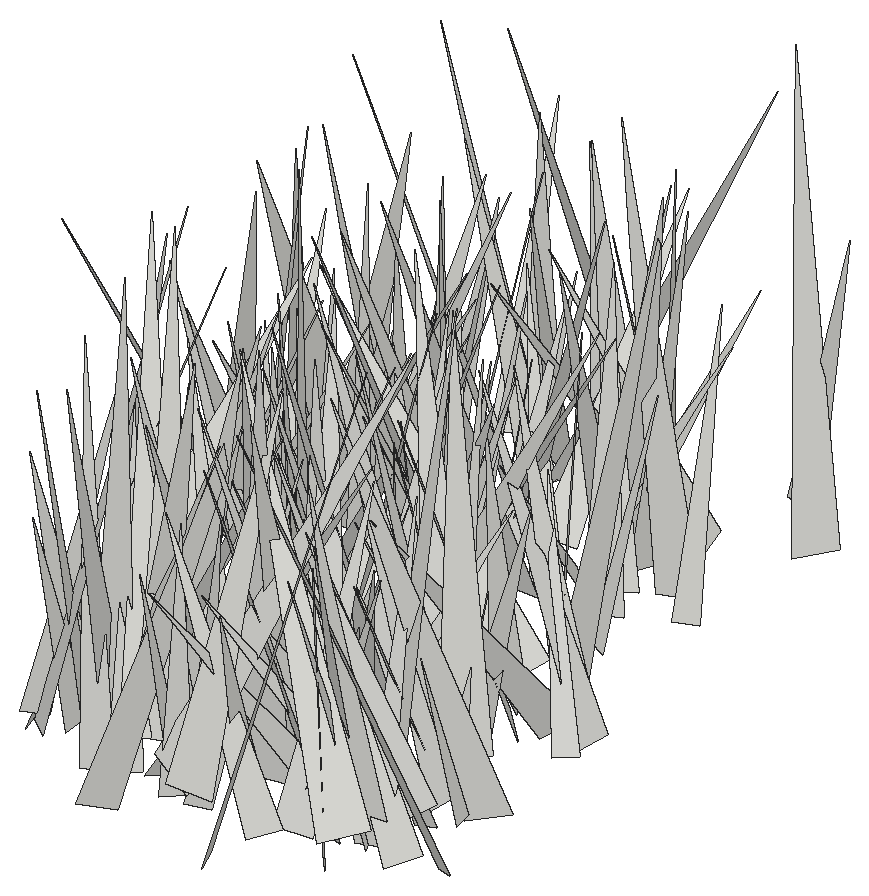
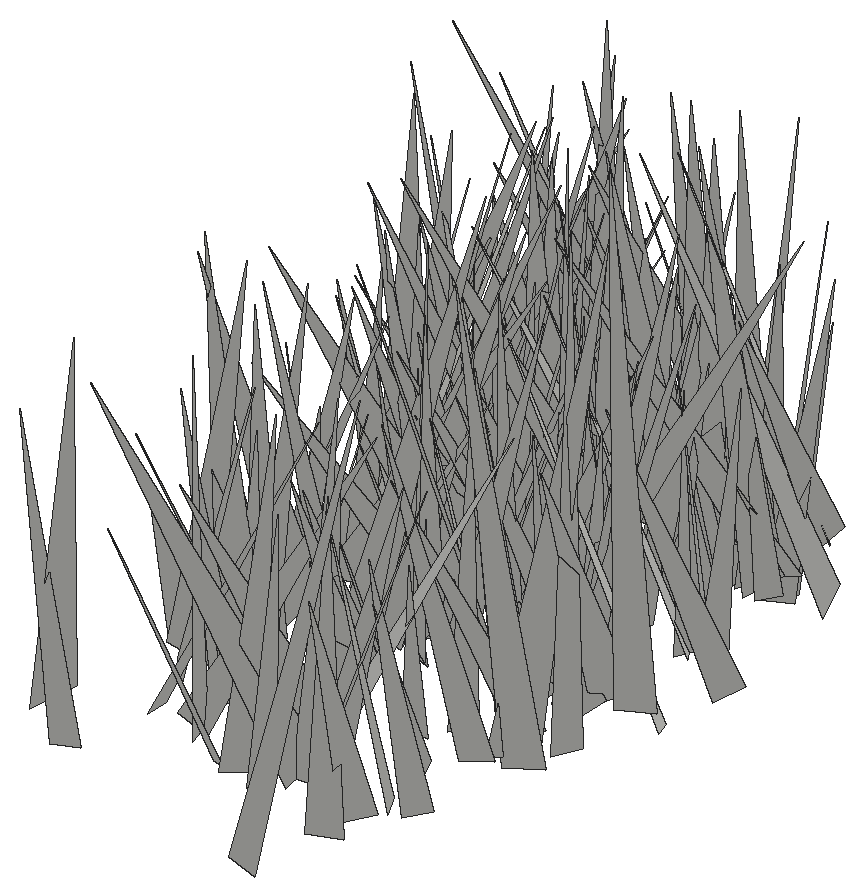
# SketchUp Ruby script. Lengths in inches.
U = 1.inch
M = Sketchup.active_model
def pt(a) = Geom::Point3d.new(a.map { |v| v * U })
def face(e, loops, mat)
  f = e.add_face(loops[0].map { |a| pt(a) })
  loops[1..].each { |l| e.add_face(l.map { |a| pt(a) }).erase! }
  f.material = f.back_material = mat if mat
  f
end
# faces: each face lists its corners as indices into pts; further lists are holes
def faces(e, pts, list, mat = nil) = list.each { |f| face(e, (f[0].is_a?(Array) ? f : [f]).map { |l| l.map { |i| pts[i] } }, mat) }
# xy, xz, yz: faces in a plane at the given z, y or x. An outline is a flat list of corners, or four numbers for a rectangle; further outlines are holes
def ring(l) = l.size == 4 ? [[l[0], l[1]], [l[2], l[1]], [l[2], l[3]], [l[0], l[3]]] : l.each_slice(2).to_a
def flat(e, list, mat, &to3) = list.each { |f| face(e, (f[0].is_a?(Array) ? f : [f]).map { |l| ring(l).map { |u, v| to3.(u, v) } }, mat) }
def xy(e, z, list, mat = nil) = flat(e, list, mat) { |x, y| [x, y, z] }
def xz(e, y, list, mat = nil) = flat(e, list, mat) { |x, z| [x, y, z] }
def yz(e, x, list, mat = nil) = flat(e, list, mat) { |y, z| [x, y, z] }
def lines(e, pts, list) = list.each { |a, b| e.add_line(pt(pts[a]), pt(pts[b])) }
# prism: a flat outline (further loops are holes) pulled along v
def prism(e, loops, v, mat = nil)
  f = face(e, loops, mat); d = Geom::Vector3d.new(v.map { |x| x * U })
  f.pushpull(f.normal.samedirection?(d) ? d.length : -d.length)
end
def box(e, o, s, mat = nil) = prism(e, [[o, [o[0] + s[0], o[1], o[2]], [o[0] + s[0], o[1] + s[1], o[2]], [o[0], o[1] + s[1], o[2]]]], [0, 0, s[2]], mat)
def at(x, y, z, deg = 0) = Geom::Transformation.translation(pt([x, y, z])) * Geom::Transformation.rotation(ORIGIN, Z_AXIS, deg.degrees)
def axes(o, x, y, z) = Geom::Transformation.new([*x, 0, *y, 0, *z, 0, *pt(o).to_a, 1])
def part(name) = M.definitions.add(name)
# library, detail: a bought-in or finely detailed component or shape, given as its bounding box
def library(name, o, s) = part(name).tap { |d| box(d.entities, o, s) }
def detail(e, o, s) = box(e.add_group.entities, o, s)
def put(e, d, t, mat = nil) = e.add_instance(d, t).tap { |i| i.material = mat if mat }
def group(e, t, mat = nil) = e.add_group.tap { |g| g.transformation = t; g.material = mat if mat }.entities
root = M.entities
c1 = part("fur_instance\#9")
p = [[0.8125,0,1.79],[0.67,-0.02,1.48],[0,-0.11,0],[0,0.11,0]]
faces(c1.entities,p,[[0,1,2,3]])
put(root,c1,axes([77.15,203.18,-28.22],[-4.827,3.94667,0.05385],[3.76525,4.62978,-1.80751],[1.18405,1.36675,5.96733]))
put(root,c1,axes([74.625,200.86,-28.22],[4.25693,-2.37845,0.80532],[-2.50825,-3.95225,1.586],[0.11926,1.77474,4.61119]))
put(root,c1,axes([74.94,208.11,-27.1],[7.73874,0.04549,1.82687],[0.5794,-7.60007,-2.26513],[-1.73315,-2.33761,7.39995]))
put(root,c1,axes([75.98,209.39,-27.1],[6.63906,-4.24471,1.17982],[-3.75911,-6.57064,-2.48644],[-2.29753,-1.51516,7.47745]))
put(root,c1,axes([76.89,193.25,-27.1],[-5.00496,1.9066,1.35129],[1.19771,4.83542,-2.3864],[2.00664,1.8693,4.79477]))
put(root,c1,axes([76.36,199.49,-28.22],[2.8154,-3.04723,0.70248],[-2.99803,-2.89898,-0.55973],[-0.88933,0.126,4.11081]))
put(root,c1,axes([77.24,215.06,-27.1],[-3.56448,3.67904,0.44666],[3.56023,3.5714,-1.00507],[1.02934,0.38746,5.02301]))
put(root,c1,axes([75.96,201.34,-27.1],[3.91592,-0.46866,0.80636],[-0.26131,-3.89224,-0.99321],[-0.89531,-0.91384,3.81675]))
put(root,c1,axes([76.02,199.99,-28.22],[3.95435,2.54343,1.52337],[2.80761,-4.0284,-0.56212],[-0.95239,-1.31514,4.66797]))
put(root,c1,axes([76.04,213.79,-27.1],[2.99214,-2.75371,1.44433],[-3.06357,-2.95389,0.71483],[-0.53251,1.52102,4.0031]))
put(root,c1,axes([77.03,195.6,-28.22],[3.57581,-3.48366,1.446],[-3.33217,-3.85124,-1.03819],[-1.76733,0.21279,4.88308]))
put(root,c1,axes([76.11,197.11,-27.1],[3.13443,-2.25979,0.73802],[-2.32723,-3.16608,0.18952],[-0.4851,0.5876,3.85946]))
put(root,c1,axes([80.1,201.87,-27.1],[-3.80092,-6.72254,0.0507],[-6.48684,3.65215,-2.05545],[-1.76524,1.05421,7.4441]))
put(root,c1,axes([74.91,204.93,-27.1],[-0.13317,-8.12567,1.45261],[-7.87911,0.55826,2.40046],[2.46092,1.34765,7.76415]))
put(root,c1,axes([80.11,213.3,-27.1],[-6.83624,-2.0461,0.45627],[-2.08301,6.45462,-2.26447],[-0.23611,2.29788,6.76704]))
put(root,c1,axes([77.03,195.1,-28.22],[3.88583,-1.17381,1.38743],[-0.79486,-4.04284,-1.19419],[-1.63432,-0.82466,3.87962]))
put(root,c1,axes([77.62,194.7,-27.1],[-4.6895,-2.45579,1.69505],[-2.43913,4.97359,0.45768],[1.71894,0.35769,5.27378]))
put(root,c1,axes([77.49,211.6,-27.1],[3.33394,1.47543,1.26624],[0.9738,-3.44268,1.44745],[-1.68284,0.93087,3.34618]))
put(root,c1,axes([75.34,209.65,-27.1],[0.9927,-7.18833,2.00129],[-7.23058,-0.4281,2.04891],[1.84279,2.19257,6.96128]))
put(root,c1,axes([81.21,210.83,-27.1],[-6.43148,-3.95381,0.27263],[-3.76371,5.93049,-2.78112],[-1.24153,2.50351,7.01869]))
put(root,c1,axes([76.65,196.6875,-27.1],[7.07212,-1.1156,2.41076],[-1.38462,-7.39913,0.63784],[-2.26697,1.03896,7.1311]))
put(root,c1,axes([79.22,193.26,-28.22],[0.02975,6.47261,1.15989],[6.34372,-0.33363,1.69906],[-1.73125,-1.11127,6.2457]))
put(root,c1,axes([77.39,216.53,-27.1],[1.77747,-4.94769,1.74658],[-5.22789,-1.82695,0.145],[-0.44649,1.69476,5.25529]))
put(root,c1,axes([78.15,205.01,-27.1],[0.81104,4.54834,1.26147],[4.65262,-0.98593,0.56355],[-0.7949,-1.13006,4.58559]))
put(root,c1,axes([79.71,201.18,-28.22],[-6.68615,-0.01766,0.93467],[0.01232,6.74773,0.2156],[0.93476,-0.21523,6.6827]))
put(root,c1,axes([78.14,219.46,-27.1],[-2.86218,-6.85746,0.77217],[-6.83354,2.93291,0.71683],[0.96112,0.43167,7.39614]))
put(root,c1,axes([78.36,203.05,-27.1],[-4.55771,-1.35516,1.4154],[-1.26006,4.77117,0.51063],[1.50069,-0.10962,4.72742]))
put(root,c1,axes([77.54,192.62,-27.1],[5.51307,6.12337,0.96272],[5.81555,-5.55551,2.03274],[-2.14519,0.67601,7.98483]))
put(root,c1,axes([76.74,208.48,-27.1],[1.64053,-3.56149,0.70323],[-3.59089,-1.47867,0.88831],[0.53314,0.99969,3.81922]))
put(root,c1,axes([76.97,213.89,-27.1],[4.26525,2.34746,1.0733],[2.44325,-4.34035,-0.2164],[-0.83252,-0.71113,4.86375]))
put(root,c1,axes([75.79,194.58,-28.22],[7.5502,3.19495,0.69372],[3.12341,-7.56468,0.84526],[-0.96605,0.51231,8.15468]))
put(root,c1,axes([76.69,210.18,-27.1],[-0.20342,5.45726,1.92359],[5.57072,0.70526,-1.41173],[1.56492,-1.80117,5.27542]))
put(root,c1,axes([79.24,201.59,-27.1],[-4.35702,1.54483,0.37411],[1.45493,4.3157,-0.87633],[0.64002,0.7059,4.53896]))
put(root,c1,axes([75.96,201.09,-27.1],[4.98455,3.49636,0.32674],[3.50629,-4.92427,-0.79656],[0.19289,-0.83908,6.03621]))
put(root,c1,axes([78.7,203.74,-28.22],[-4.7956,1.01448,1.55419],[0.95492,5.04106,-0.34401],[1.59148,0.0322,4.88965]))
put(root,c1,axes([78.79,198.26,-27.1],[-3.8802,0.07929,1.10053],[0.11582,4.03064,0.11798],[1.09728,-0.14508,3.87922]))
put(root,c1,axes([77.84,204.24,-28.22],[6.61822,-2.56323,1.80089],[-1.74555,-6.51281,-2.85492],[-2.60123,-2.15113,6.49773]))
put(root,c1,axes([74.86,203.72,-28.22],[5.8637,3.4963,0.04079],[3.31459,-5.53283,-2.23832],[1.11324,-1.94227,6.44958]))
put(root,c1,axes([76.23,208.14,-27.1],[4.34648,-1.55951,0.20323],[-1.53377,-4.07129,1.56122],[0.34774,1.53551,4.34586]))
put(root,c1,axes([79.76,213.33,-27.1],[0.51311,-4.91857,2.52241],[-5.22585,-1.25725,-1.38854],[-1.80151,2.24614,4.74633]))
put(root,c1,axes([79.17,210.01,-27.1],[-0.87591,3.86506,0.33078],[3.84564,0.82067,0.59405],[-0.50909,-0.4507,3.91829]))
put(root,c1,axes([76.67,195.89,-27.1],[-0.73588,7.38124,0.25307],[6.98236,0.77818,-2.39362],[2.40696,-0.00075,7.02103]))
put(root,c1,axes([78.65,201.09,-27.1],[5.2038,5.70361,2.35891],[5.67233,-5.63566,1.11317],[-2.43315,-0.93989,7.64013]))
put(root,c1,axes([78.25,208.86,-27.1],[4.81176,-1.3762,1.70282],[-1.26945,-5.10354,-0.53746],[-1.78382,-0.0803,4.97575]))
put(root,c1,axes([80.67,206.27,-27.1],[-3.32037,-5.8988,2.51801],[-6.36421,2.67847,-2.11746],[-0.7956,3.19234,6.42939]))
put(root,c1,axes([77.15,207.62,-27.1],[2.1882,-4.93746,0.79161],[-4.93819,-1.99768,1.19031],[0.78701,1.19336,5.26781]))
put(root,c1,axes([79.8125,204.48,-27.1],[1.26749,-5.25605,0.55346],[-5.00773,-1.37633,-1.60227],[-1.68968,0.13629,5.16385]))
put(root,c1,axes([78.76,194.54,-27.1],[-0.16128,6.84934,2.86842],[7.42417,0.20732,-0.07764],[0.15166,-2.86546,6.8508]))
put(root,c1,axes([78.35,195.32,-28.22],[6.75782,0.35235,2.65885],[1.16075,-6.88187,-2.03823],[-2.41791,-2.31896,6.45275]))
put(root,c1,axes([78.65,202.73,-28.22],[0.54293,-5.17192,1.62827],[-5.42158,-0.49338,0.24063],[0.08095,1.64396,5.19477]))
put(root,c1,axes([79.98,193.61,-28.22],[-5.05186,2.37101,0.85511],[2.22237,5.09377,-0.9944],[1.18912,0.55319,5.49128]))
put(root,c1,axes([80.45,194.16,-27.1],[-5.1988,6.07272,1.14347],[6.1224,5.26442,-0.12263],[0.83765,-0.78798,7.99315]))
put(root,c1,axes([79.75,199.91,-27.1],[-0.43977,4.5707,0.64422],[4.59918,0.3789,0.45132],[-0.39225,-0.6818,4.56957]))
put(root,c1,axes([77.23,204.14,-28.22],[5.25696,-1.00652,0.21452],[-1.02902,-5.15697,1.02054],[-0.01477,1.04274,5.25426]))
put(root,c1,axes([79.34,203.57,-28.22],[-4.01189,-2.17426,1.82805],[-1.57492,4.33524,1.69992],[2.36407,-0.80168,4.23473]))
put(root,c1,axes([80.69,197.24,-28.22],[-6.42976,0.15301,2.02637],[0.5172,6.6259,1.14077],[1.96522,-1.24316,6.3296]))
put(root,c1,axes([79.31,199.2,-28.22],[6.21031,-0.46369,2.15458],[0.49806,-5.98034,-2.72263],[-2.14689,-2.7287,5.60092]))
put(root,c1,axes([77.81,198.61,-27.1],[4.01839,-5.64573,1.18023],[-5.73753,-3.76564,1.52164],[0.58986,1.83314,6.76065]))
put(root,c1,axes([80.7,203.59,-27.1],[1.55743,6.34801,1.89562],[6.44853,-1.89902,1.06134],[-1.51893,-1.55328,6.44953]))
put(root,c1,axes([80.83,194.28,-27.1],[-1.87564,7.62096,1.95831],[7.8685,1.80971,0.49369],[-0.027,-2.0194,7.83284]))
put(root,c1,axes([80.94,215.03,-27.1],[-4.87312,1.26006,1.29377],[1.19613,5.04128,-0.40455],[1.35309,0.08157,5.01711]))
put(root,c1,axes([80.02,205.14,-28.22],[3.87453,3.49507,1.24049],[3.40824,-4.0629,0.80191],[-1.46226,-0.20898,5.15601]))
put(root,c1,axes([77.35,207.51,-27.1],[5.13352,5.29295,1.04527],[5.31008,-4.70157,-2.27141],[0.95446,-2.31104,7.01492]))
put(root,c1,axes([82.11,195.86,-27.1],[-1.56415,5.71782,0.81541],[5.62888,1.31989,1.54221],[-1.29382,-1.17019,5.72377]))
put(root,c1,axes([78.37,194.38,-28.22],[4.45392,4.12687,0.87812],[4.21021,-4.26347,-1.31776],[0.27618,-1.55927,5.92722]))
put(root,c1,axes([81.2,208.52,-27.1],[1.74005,3.73475,0.21366],[3.48509,-1.70407,1.40429],[-1.35946,0.41179,3.87351]))
put(root,c1,axes([79.9,214.31,-27.1],[-1.23587,-5.65616,0.92472],[-5.5483,1.41785,1.25724],[1.43652,0.61007,5.65145]))
put(root,c1,axes([79,197.01,-28.22],[2.95876,-6.29379,1.88961],[-6.54545,-2.63888,1.45948],[0.58268,2.31543,6.79971]))
put(root,c1,axes([79.36,195.58,-27.1],[2.15737,-6.51602,1.69287],[-6.69271,-1.88316,1.28061],[0.7294,1.99342,6.74336]))
put(root,c1,axes([78.65,195.47,-28.22],[6.19791,-1.23637,0.25272],[-1.26158,-6.10069,1.0939],[-0.02993,1.12232,6.22464]))
put(root,c1,axes([80.58,191.56,-28.22],[7.42059,-0.17453,3.00871],[-1.57677,-7.03899,3.48057],[-2.56838,3.81708,6.55601]))
put(root,c1,axes([79.36,202.89,-27.1],[5.44463,0.12063,0.24069],[0.04962,-5.23956,1.50366],[-0.26462,1.49964,5.23426]))
put(root,c1,axes([81.47,194.28,-28.22],[-0.47471,-3.8388,0.84095],[-3.92781,0.49062,0.02236],[0.12592,0.83177,3.86797]))
put(root,c1,axes([82.68,198.67,-27.1],[-7.45834,-2.27512,2.73301],[-2.96816,7.48025,-1.87304],[1.95846,2.67246,7.56933]))
put(root,c1,axes([81.73,215.04,-27.1],[3.82096,-4.05561,2.24215],[-4.19487,-4.26194,-0.56033],[-1.96935,1.20949,5.5438]))
put(root,c1,axes([82.61,204.93,-27.1],[-6.55431,0.09701,1.7896],[-0.34688,6.588,-1.62754],[1.75834,1.66126,6.34976]))
put(root,c1,axes([79.92,200.45,-28.22],[0.34985,-8.1007,0.677],[-7.9597,-0.20383,1.67442],[1.6501,0.73429,7.93347]))
put(root,c1,axes([82.14,202,-27.1],[0.37183,-3.94608,0.38846],[-3.8933,-0.43727,-0.71534],[-0.75144,0.31297,3.89847]))
put(root,c1,axes([80.95,201.99,-27.1],[-0.63847,4.33122,0.11328],[4.14955,0.64421,-1.24344],[1.2464,0.07394,4.19773]))
put(root,c1,axes([82.39,202.03,-27.1],[-3.37943,-0.96857,0.84627],[-0.6019,3.29348,1.36586],[1.13667,-1.13567,3.23931]))
put(root,c1,axes([82.73,198.84,-28.22],[3.81307,5.29138,3.34018],[5.75803,-4.49829,0.55278],[-2.44962,-2.33704,6.49867]))
put(root,c1,axes([81.99,193.53,-28.22],[3.33409,-2.8819,1.80128],[-3.12207,-3.59416,0.02846],[-1.34262,1.20116,4.40689]))
put(root,c1,axes([83.625,206.11,-27.1],[-0.04463,-6.97717,1.39975],[-6.92736,-0.27772,-1.60522],[-1.62845,1.37265,6.79015]))
put(root,c1,axes([82.19,206.1,-27.1],[3.78368,4.97369,3.03573],[5.56614,-4.15585,-0.12867],[-1.72376,-2.50217,6.24798]))
put(root,c1,axes([82.7,204.43,-27.1],[-2.40754,3.72637,1.88833],[4.14407,2.40561,0.53634],[0.52762,-1.89079,4.40391]))
put(root,c1,axes([83.76,201.64,-28.22],[-5.02334,-0.16728,0.55191],[-0.071,4.98153,0.86367],[0.57231,-0.85028,4.95137]))
put(root,c1,axes([83.34,196.96,-28.22],[-5.20455,-0.25594,1.25726],[-0.61037,5.11409,-1.48563],[1.12857,1.58561,4.99457]))
put(root,c1,axes([82.37,208.59,-27.1],[-4.0426,1.99311,1.15136],[1.52694,4.06338,-1.67276],[1.72237,1.07573,4.18533]))
put(root,c1,axes([83.69,208.78,-27.1],[-4.1604,2.35856,0.20079],[2.33408,4.15517,-0.44576],[0.39395,0.28953,4.76162]))
put(root,c1,axes([82.45,208.09,-27.1],[-3.28423,2.60896,0.74342],[2.31234,3.30268,-1.37511],[1.4186,0.65664,3.96257]))
put(root,c1,axes([79.5,198.96,-27.1],[7.73901,0.54751,0.09462],[0.50511,-7.48314,1.98706],[-0.23147,1.9758,7.49957]))
put(root,c1,axes([83.34,207.87,-27.1],[-0.92127,-7.60318,0.93237],[-7.64439,0.85236,-0.60268],[-0.49091,0.99576,7.63504]))
put(root,c1,axes([82.15,194.4,-27.1],[-3.43259,1.11019,2.13702],[1.24058,4.00441,-0.08763],[2.06406,-0.56053,3.60659]))
put(root,c1,axes([80.3,213.86,-27.1],[7.35163,-0.33714,0.71191],[-0.54127,-7.01692,2.26646],[-0.57229,2.30568,7.00167]))
put(root,c1,axes([82.46,210.83,-27.1],[-2.9389,4.8588,0.20427],[4.55933,2.83593,-1.85926],[1.6918,0.79774,5.36547]))
put(root,c1,axes([82.9,193.4,-28.22],[-4.89219,1.92037,1.37183],[1.09822,4.64707,-2.5888],[2.08893,2.05431,4.57377]))
put(root,c1,axes([83.9375,200.52,-28.22],[-5.80555,-2.80529,1.19859],[-2.69051,5.92298,0.83076],[1.43785,-0.24369,6.39405]))
put(root,c1,axes([84.88,205.96,-27.1],[-2.69174,-3.80387,0.07847],[-3.66679,2.56798,-1.29661],[-1.01502,0.8106,4.47591]))
put(root,c1,axes([84.63,213.68,-27.1],[0.43766,-5.35462,0.13989],[-4.92597,-0.45748,-2.09965],[-2.10387,-0.04276,4.94519]))
put(root,c1,axes([81.72,196.6,-27.1],[5.03516,3.5658,0.22039],[3.50469,-5.00395,0.89105],[-0.69327,0.6016,6.10523]))
put(root,c1,axes([86.66,204.2,-27.1],[-6.39943,2.86094,0.01202],[2.71801,6.07041,2.2137],[-0.89308,-2.0256,6.65111]))
put(root,c1,axes([80.54,203.31,-28.22],[7.66511,2.45698,1.17946],[2.70747,-7.26796,-2.45522],[-0.3122,-2.70587,7.66567]))
put(root,c1,axes([86.07,203.34,-27.1],[-4.08084,-6.31933,0.93728],[-6.28934,3.77891,-1.90517],[-1.12095,1.80323,7.27719]))
put(root,c1,axes([83.11,204.89,-28.22],[1.95636,4.4496,1.57567],[4.70552,-1.97342,-0.26957],[-0.3738,-1.55425,4.8532]))
put(root,c1,axes([83.3,198.65,-28.22],[4.24659,-4.94069,2.32668],[-5.22174,-4.53655,-0.10277],[-1.59916,1.69313,6.51409]))
put(root,c1,axes([83.4,204.21,-27.1],[1.4103,3.34023,0.25009],[3.32818,-1.428,0.30438],[-0.37801,-0.11091,3.61295]))
put(root,c1,axes([85.47,193.3,-28.22],[-3.5373,3.73043,1.14853],[3.88761,3.22863,1.48666],[-0.34887,-1.84596,4.92122]))
put(root,c1,axes([84.7,200.51,-27.1],[-5.37291,2.30629,0.61766],[1.96946,5.14098,-2.06404],[1.34972,1.6793,5.47055]))
put(root,c1,axes([81.875,209.56,-27.1],[6.64605,0.23955,0.93352],[0.28653,-6.70181,-0.32012],[-0.92019,-0.35664,6.64266]))
put(root,c1,axes([86.18,195.39,-27.1],[-5.88175,-1.50758,0.15009],[-1.51502,5.85044,-0.60606],[-0.00586,0.62434,6.04156]))
put(root,c1,axes([84.67,195.875,-27.1],[-4.21387,-1.59887,0.24339],[-1.27519,3.70248,2.24451],[0.99474,-2.02671,3.90836]))
put(root,c1,axes([84.125,202.71,-27.1],[-3.08736,-2.6391,1.38175],[-2.74426,3.29386,0.15946],[1.15895,0.7691,4.05847]))
put(root,c1,axes([80.96,194.25,-28.22],[6.564,-1.73993,0.0582],[-1.67851,-6.26496,2.01239],[0.46191,1.95953,6.48565]))
put(root,c1,axes([86.07,213.59,-27.1],[-5.4104,-1.19331,0.05848],[-1.15989,5.3113,1.06983],[0.28647,-1.03242,5.43616]))
put(root,c1,axes([85.37,199.71,-28.22],[-3.27464,-6.78559,1.40651],[-6.92909,3.22889,-0.5548],[0.10135,1.50857,7.51397]))
put(root,c1,axes([83.24,195.95,-28.22],[2.47243,-7.62212,2.09201],[-7.90302,-2.41845,0.52868],[-0.12434,2.1542,7.99563]))
put(root,c1,axes([84.95,196.57,-27.1],[-3.82919,5.78151,1.38736],[5.88668,3.91838,-0.08139],[0.83523,-1.11076,6.93412]))
put(root,c1,axes([82.56,215.0625,-27.1],[2.24479,3.42751,0.35228],[3.3467,-2.06895,-1.19586],[0.81948,-0.93948,3.91878]))
put(root,c1,axes([84.7,204.67,-28.22],[2.63198,-5.20128,0.6124],[-4.94839,-2.69423,-1.6156],[-1.71515,-0.20845,5.60093]))
put(root,c1,axes([86.08,197.52,-28.22],[-1.75901,-5.06572,0.78099],[-4.97011,1.48393,-1.5689],[-1.25276,1.22556,5.12778]))
put(root,c1,axes([83.42,192.33,-27.1],[-1.23701,6.48468,1.94316],[6.59867,1.59608,-1.12573],[1.51147,-1.6609,6.50492]))
put(root,c1,axes([83.57,202.8,-28.22],[-0.45629,-4.37673,0.42276],[-4.25435,0.54685,1.06962],[1.11127,0.29645,4.26847]))
put(root,c1,axes([83.83,194.75,-28.22],[3.81403,-1.87609,0.65313],[-1.66249,-3.78837,-1.17367],[-1.0874,-0.78844,4.08523]))
put(root,c1,axes([84.93,198.13,-27.1],[-3.91308,1.33626,1.31278],[1.41439,4.10109,0.04154],[1.2282,-0.46546,4.13474]))
put(root,c1,axes([84.16,213.91,-27.1],[5.47086,1.91538,2.35531],[2.21322,-5.83902,-0.39241],[-2.07794,-1.17628,5.78316]))
put(root,c1,axes([84.61,202.97,-27.1],[2.40837,2.51325,1.53163],[2.71206,-2.66382,0.10655],[-1.14326,-1.0248,3.47927]))
put(root,c1,axes([82.67,204.09,-27.1],[5.53562,0.75174,0.06867],[0.66774,-5.11345,2.14935],[-0.35205,2.12143,5.1564]))
put(root,c1,axes([83.97,197.19,-28.22],[5.27875,-5.42072,0.96709],[-5.29735,-5.36505,-1.15714],[-1.50251,-0.12916,7.47733]))
put(root,c1,axes([84.33,200.87,-27.1],[-3.42009,-2.62307,1.97794],[-2.56254,3.91671,0.76324],[2.05575,0.51835,4.24205]))
put(root,c1,axes([84.38,209.48,-27.1],[-2.58943,-3.13022,0.07236],[-2.65217,2.2427,2.10831],[1.66419,-1.2964,3.47253]))
put(root,c1,axes([87.3,194.34,-28.22],[-3.98273,-4.40716,0.90523],[-4.3967,3.55588,-2.0321],[-0.95477,2.0093,5.58174]))
put(root,c1,axes([85.9375,204.48,-28.22],[-5.99255,-5.60768,0.41861],[-5.37957,5.89507,1.95969],[1.63755,-1.155,7.96972]))
put(root,c1,axes([83.77,198.5625,-27.1],[6.82922,2.21825,1.16198],[1.82522,-6.72015,2.10172],[-1.71447,1.68168,6.86597]))
put(root,c1,axes([84.6,210.83,-27.1],[0.33482,-6.22736,0.74708],[-6.26175,-0.28913,0.39628],[0.3585,0.76592,6.22375]))
put(root,c1,axes([82.17,204.82,-27.1],[1.01842,-6.5564,0.3467],[-5.92672,-0.76709,2.90332],[2.82498,0.75429,5.9661]))
put(root,c1,axes([84.44,199.3,-27.1],[-2.07384,5.25709,1.74566],[5.26815,2.4479,-1.11335],[1.712,-1.16445,5.54061]))
put(root,c1,axes([86.35,196.22,-27.1],[-4.14982,-0.72477,0.23143],[-0.53834,3.70403,1.94686],[0.53763,-1.88541,3.73578]))
put(root,c1,axes([85.84,209.65,-27.1],[-2.17723,3.86998,1.04919],[4.00343,2.16477,0.32287],[0.22393,-1.07466,4.42864]))
put(root,c1,axes([85.44,211.12,-27.1],[5.18015,0.30458,2.40247],[-0.20645,-5.59667,1.15468],[-2.41288,1.13276,5.059]))
put(root,c1,axes([82.3125,192.85,-27.1],[2.96543,7.80813,0.73471],[7.53088,-2.61577,-2.59693],[2.18919,-1.57838,7.9383]))
put(root,c1,axes([86.94,211.41,-27.1],[-4.01127,-3.66818,1.32519],[-3.89401,3.87381,-1.06408],[0.2199,1.68524,5.33044]))
put(root,c1,axes([84.64,201.0625,-27.1],[4.97283,-0.90694,1.68915],[-1.45035,-4.85051,1.66547],[-1.25389,2.01364,4.77261]))
put(root,c1,axes([85.6,202.66,-28.22],[-3.75985,-4.2409,1.14983],[-3.97997,3.92819,1.47409],[1.86202,-0.16705,5.47255]))
put(root,c1,axes([85,202.72,-28.22],[3.25628,-4.96201,1.27437],[-5.08219,-3.31911,0.06246],[-0.64574,1.10043,5.93473]))
put(root,c1,axes([88.42,198.38,-28.22],[-8.26176,0.40654,0.83522],[0.41692,8.30295,0.08258],[0.83009,-0.12394,8.27135]))
put(root,c1,axes([84.25,211.62,-27.1],[4.71855,-5.46855,1.25045],[-5.59838,-4.69426,0.59612],[-0.35606,1.33873,7.19821]))
put(root,c1,axes([88.63,193.08,-27.1],[-6.09178,4.42452,0.24879],[4.41982,6.03543,0.88707],[-0.32169,-0.86331,7.47659]))
put(root,c1,axes([83.72,211.11,-27.1],[2.80072,3.68056,0.20092],[3.50306,-2.57922,-1.58339],[1.14693,-1.10998,4.34551]))
put(root,c1,axes([87.33,210.45,-27.1],[-0.80473,7.1427,2.6366],[7.51279,0.31449,1.44102],[-1.23607,-2.73867,7.04196]))
put(root,c1,axes([85.12,191.02,-28.22],[6.6915,4.26773,1.20587],[3.94044,-6.72308,1.92792],[-2.03484,1.01512,7.69888]))
put(root,c1,axes([83.79,201.72,-27.1],[5.89458,-2.32049,1.52507],[-2.76984,-5.16651,2.8446],[-0.1962,3.22166,5.6603]))
put(root,c1,axes([87.43,200.92,-28.22],[-4.15133,-1.53142,0.10873],[-1.49707,4.10736,0.69206],[0.34034,-0.61232,4.37033]))
put(root,c1,axes([86.23,208.23,-27.1],[-2.39493,4.93051,2.15105],[5.27679,2.61079,-0.10925],[1.04521,-1.88321,5.4803]))
put(root,c1,axes([88.18,196.6875,-28.22],[-6.23663,-1.3966,0.55844],[-1.37103,6.25805,0.33911],[0.61857,-0.21031,6.38209]))
put(root,c1,axes([87.82,199.2,-27.1],[-6.04844,4.67756,1.28768],[4.75602,6.12308,0.0974],[0.95811,-0.86582,7.6455]))
put(root,c1,axes([89.67,194.58,-28.22],[-2.08516,6.03207,0.25096],[5.29839,1.7011,3.1353],[-2.89412,-1.23172,5.5591]))
put(root,c1,axes([86.01,193.96,-28.22],[-1.65909,5.33475,1.21269],[5.33342,1.85943,-0.88312],[1.21852,-0.87506,5.51654]))
put(root,c1,axes([86.95,200.48,-28.22],[4.44395,3.96646,1.43413],[3.47391,-4.62357,2.02305],[-2.39195,0.65422,5.60257]))
put(root,c1,axes([87.1,203,-28.22],[-4.26482,-5.03014,0.77761],[-4.82923,4.31941,1.45497],[1.60794,-0.36894,6.43227]))
put(root,c1,axes([85.1,198.13,-28.22],[5.22724,-1.35677,0.09683],[-1.28473,-5.05093,-1.4184],[-0.44684,-1.34966,5.21086]))
put(root,c1,axes([86.66,203.25,-27.1],[3.6689,-2.8215,1.45683],[-2.81207,-3.92099,-0.512],[-1.47496,0.45716,4.59995]))
put(root,c1,axes([84.95,197.88,-28.22],[2.06268,4.77096,0.10661],[4.57909,-1.94603,-1.50762],[1.34363,-0.69206,4.97431]))
put(root,c1,axes([88.38,203.29,-28.22],[3.82585,4.29132,1.89582],[3.55577,-4.24822,2.44044],[-3.06039,0.42878,5.20545]))
put(root,c1,axes([88.5,204.26,-28.22],[-5.29366,2.0126,1.17564],[2.12712,5.36423,0.39489],[0.95291,-0.79376,5.64955]))
put(root,c1,axes([89.56,203.65,-28.22],[-5.92651,0.06077,0.05927],[0.05827,5.92175,-0.24529],[0.06173,0.24468,5.92174]))
put(root,c1,axes([88.86,214.99,-27.1],[-7.32985,2.37013,1.25415],[2.21242,7.40801,-1.06942],[1.51512,0.64882,7.62892]))
put(root,c1,axes([86.28,194.77,-27.1],[3.72364,-1.08643,0.80362],[-1.21362,-3.72465,0.58799],[-0.59435,0.79892,3.83407]))
put(root,c1,axes([89.43,197.86,-28.22],[-7.02647,-2.17808,1.10616],[-2.29777,7.03636,-0.74079],[0.82938,1.04138,7.31892]))
put(root,c1,axes([87.67,204.68,-28.22],[7.23662,0.86237,3.59764],[-0.54989,-7.56504,2.91946],[-3.65846,2.84288,6.67751]))
put(root,c1,axes([88.47,209.35,-27.1],[-4.48023,1.71415,0.10108],[1.53614,4.12726,-1.90446],[0.76734,1.74596,4.4027]))
put(root,c1,axes([88.37,198.53,-27.1],[1.19098,5.93826,0.851],[5.76454,-1.37303,1.51343],[-1.66049,-0.50738,5.86438]))
put(root,c1,axes([88.39,194.82,-28.22],[0.19192,-5.71021,2.24229],[-6.02696,-0.59408,-0.99702],[-1.14462,2.17066,5.62577]))
put(root,c1,axes([88.83,196.68,-28.22],[-0.99125,-4.30354,0.98962],[-4.28593,0.69339,-1.27766],[-1.06332,1.21702,4.22737]))
put(root,c1,axes([88.04,195.04,-28.22],[-4.22717,-2.44585,1.01456],[-2.28976,4.33627,0.91336],[1.32985,-0.3083,4.79759]))
put(root,c1,axes([90.99,194.86,-28.22],[-4.75874,-5.64309,0.42264],[-5.39038,4.3522,-2.58279],[-1.72245,1.97043,6.91515]))
put(root,c1,axes([88.26,203.68,-28.22],[3.78174,-4.82109,0.17581],[-4.12071,-3.34423,-3.06777],[-2.50869,-1.77444,5.30408]))
put(root,c1,axes([88.14,195.41,-27.1],[0.35019,4.61175,0.40741],[4.56098,-0.41379,0.76359],[-0.79477,-0.34263,4.56155]))
put(root,c1,axes([87.83,193.14,-28.22],[3.3067,2.95122,2.18217],[3.23124,-3.73382,0.15332],[-1.74087,-1.32466,4.4295]))
put(root,c1,axes([87.29,199.07,-28.22],[-2.3415,-4.6423,0.1365],[-4.37976,2.25803,1.66471],[1.54509,-0.63449,4.92568]))
put(root,c1,axes([86.75,195.72,-27.1],[-1.94792,-5.41513,0.85515],[-5.11405,2.12183,1.78705],[1.97517,0.15336,5.47032]))
put(root,c1,axes([87.33,206.59,-27.1],[1.79566,3.71313,0.76849],[3.77743,-1.82574,-0.00496],[-0.33004,-0.69403,4.12452]))
put(root,c1,axes([89.98,198.23,-28.22],[1.0703,-6.74535,2.51722],[-6.58595,-1.94546,-2.41292],[-2.90886,1.9228,6.3893]))
put(root,c1,axes([88.39,199.09,-27.1],[-4.52139,5.22079,2.42729],[5.56937,4.74843,0.161],[1.45961,-1.94607,6.90462]))
put(root,c1,axes([87.78,196.04,-28.22],[3.67219,7.15908,2.03524],[7.27938,-3.92759,0.68132],[-1.55086,-1.48365,8.01705]))
put(root,c1,axes([89.44,195.66,-27.1],[-4.32688,2.05759,1.06704],[2.30248,4.07514,1.47851],[0.2661,-1.80382,4.55737]))
put(root,c1,axes([86.77,217.04,-27.1],[0.64184,-5.02818,1.67754],[-5.1921,-0.25617,1.21871],[1.0672,1.77778,4.9203]))
put(root,c1,axes([89.47,202.47,-28.22],[-1.23895,4.11427,0.01816],[3.97981,1.19363,1.09497],[-1.04341,-0.33255,4.15491]))
put(root,c1,axes([86.73,201.51,-28.22],[3.32524,-3.2763,0.88677],[-3.39381,-3.22791,0.80025],[-0.05063,1.1934,4.59902]))
